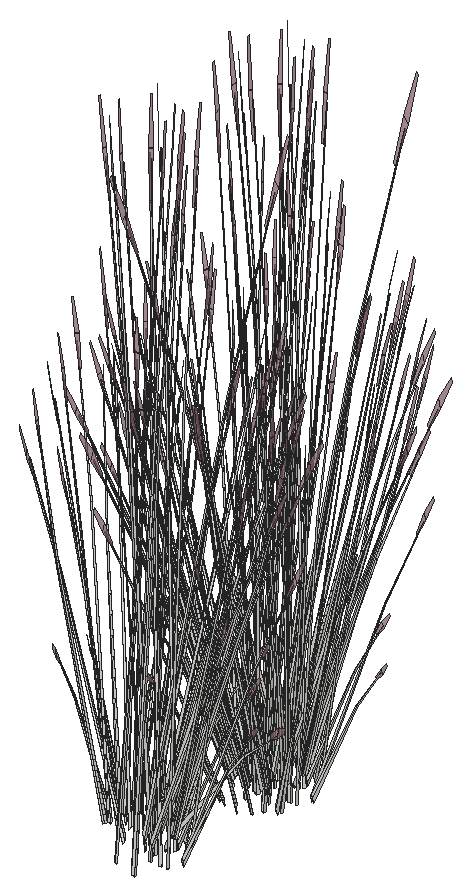
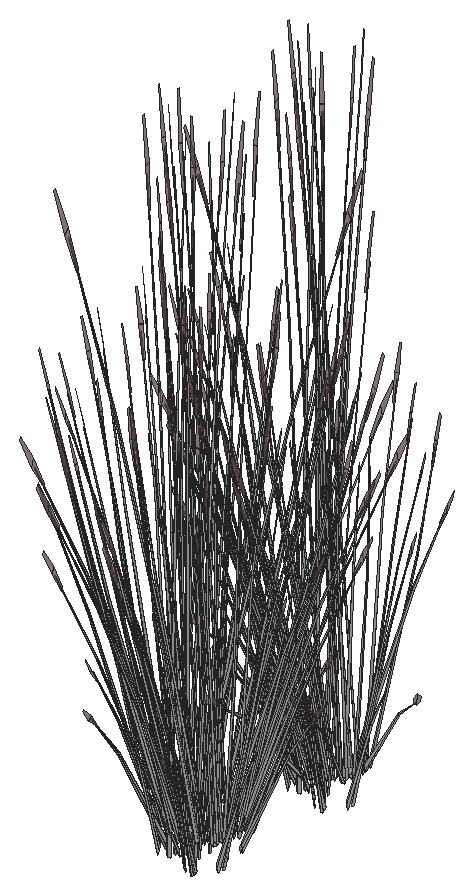
# SketchUp Ruby script. Lengths in inches.
U = 1.inch
M = Sketchup.active_model
def pt(a) = Geom::Point3d.new(a.map { |v| v * U })
def face(e, loops, mat)
  f = e.add_face(loops[0].map { |a| pt(a) })
  loops[1..].each { |l| e.add_face(l.map { |a| pt(a) }).erase! }
  f.material = f.back_material = mat if mat
  f
end
# faces: each face lists its corners as indices into pts; further lists are holes
def faces(e, pts, list, mat = nil) = list.each { |f| face(e, (f[0].is_a?(Array) ? f : [f]).map { |l| l.map { |i| pts[i] } }, mat) }
# xy, xz, yz: faces in a plane at the given z, y or x. An outline is a flat list of corners, or four numbers for a rectangle; further outlines are holes
def ring(l) = l.size == 4 ? [[l[0], l[1]], [l[2], l[1]], [l[2], l[3]], [l[0], l[3]]] : l.each_slice(2).to_a
def flat(e, list, mat, &to3) = list.each { |f| face(e, (f[0].is_a?(Array) ? f : [f]).map { |l| ring(l).map { |u, v| to3.(u, v) } }, mat) }
def xy(e, z, list, mat = nil) = flat(e, list, mat) { |x, y| [x, y, z] }
def xz(e, y, list, mat = nil) = flat(e, list, mat) { |x, z| [x, y, z] }
def yz(e, x, list, mat = nil) = flat(e, list, mat) { |y, z| [x, y, z] }
def lines(e, pts, list) = list.each { |a, b| e.add_line(pt(pts[a]), pt(pts[b])) }
# prism: a flat outline (further loops are holes) pulled along v
def prism(e, loops, v, mat = nil)
  f = face(e, loops, mat); d = Geom::Vector3d.new(v.map { |x| x * U })
  f.pushpull(f.normal.samedirection?(d) ? d.length : -d.length)
end
def box(e, o, s, mat = nil) = prism(e, [[o, [o[0] + s[0], o[1], o[2]], [o[0] + s[0], o[1] + s[1], o[2]], [o[0], o[1] + s[1], o[2]]]], [0, 0, s[2]], mat)
def at(x, y, z, deg = 0) = Geom::Transformation.translation(pt([x, y, z])) * Geom::Transformation.rotation(ORIGIN, Z_AXIS, deg.degrees)
def axes(o, x, y, z) = Geom::Transformation.new([*x, 0, *y, 0, *z, 0, *pt(o).to_a, 1])
def part(name) = M.definitions.add(name)
# library, detail: a bought-in or finely detailed component or shape, given as its bounding box
def library(name, o, s) = part(name).tap { |d| box(d.entities, o, s) }
def detail(e, o, s) = box(e.add_group.entities, o, s)
def put(e, d, t, mat = nil) = e.add_instance(d, t).tap { |i| i.material = mat if mat }
def group(e, t, mat = nil) = e.add_group.tap { |g| g.transformation = t; g.material = mat if mat }.entities
root = M.entities
M.materials.add("LightPink_Translucent").color = [144, 107, 117]
M.materials["LightPink_Translucent"].alpha = 0.75
c1 = part("blade")
p = [[2.15,0.21,22],[0,0.17,0],[0.09,0.45,0],[2.18,0.31,22],[2.29,0.31,22],[0.38,0.45,0],
  [2.48,0.24,33],[2.49,0.24,33],[2.48,0.22,33]]
faces(c1.entities,p,[[0,1,2,3],[4,5,2,3],[6,3,4,7],[8,0,3,6]])
c2 = part("seeds")
p = [[0.3,-0.1,1.38],[-0.01,-0.03,1.59],[-0.01,-0.03,0.03],[0.14,-0.07,-0.07],[0.29,-0.03,3],[0.15,0.01,3.11]]
faces(c2.entities,p,[[0,1,2,3],[1,0,4,5]],"LightPink_Translucent")
c3 = part("blade with seeds")
put(c3.entities,c1,at(0,0,0))
put(c3.entities,c2,axes([2.4,0.25,30.99],[1.5799,-0.05474,1.17369],[-0.12525,1.92788,0.29478],[-0.07173,-0.02425,1.56792]))
put(root,c3,axes([372.04,325.99,152.33],[-0.4583,-0.30184,0.46672],[0.27394,-0.54125,0],[0.10438,0.06875,1.48054]))
put(root,c3,axes([372.94,328.11,154.68],[0.4303,-0.26662,-0.66783],[0.23981,0.54882,0.08059],[0.20791,-0.06234,0.9447]))
put(root,c3,axes([370.31,326.27,152.33],[-0.14146,0.59996,0.16584],[-0.51766,-0.16978,0.32981],[0.08942,-0.00292,1.50782]))
put(root,c3,axes([371.19,327.07,152.56],[-0.29417,-0.5067,0.42055],[0.44558,-0.35681,-0.2024],[0.0952,0.0627,1.35025]))
put(root,c3,axes([370.26,329.36,152.33],[0.52621,-0.16023,0.16584],[0.12993,0.59629,0.32981],[-0.04693,-0.08688,1.50782]))
put(root,c3,axes([373.31,328.16,154.25],[0.40696,0.16841,-0.33289],[-0.1187,0.49132,0.42977],[0.16385,-0.04505,0.82232]))
put(root,c3,axes([368.52,327.38,154.25],[-0.40696,-0.16841,-0.33289],[0.1187,-0.49132,0.42977],[-0.16385,0.04505,0.82232]))
put(root,c3,axes([371.87,326.3,152.33],[-0.52621,0.16023,0.16584],[-0.12993,-0.59629,0.32981],[0.04693,0.08688,1.50782]))
put(root,c3,axes([372.2,327.56,153.64],[-0.20312,0.01367,1.61094],[0.13474,-0.59258,0.13026],[0.28946,0.03665,0.68866]))
put(root,c3,axes([370.74,328.73,152.46],[-0.09447,0.53876,0.13611],[-0.46155,-0.09352,-0.38866],[-0.084,-0.05532,1.1914]))
put(root,c3,axes([371.82,329.39,152.33],[0.14146,-0.59996,0.16584],[0.51766,0.16978,0.32981],[-0.08942,0.00292,1.50782]))
put(root,c3,axes([369.76,327.3,153.14],[0.13919,-0.08733,1.6644],[0.048,0.60974,0.13026],[-0.3015,0.08091,0.59487]))
put(root,c3,axes([372.63,327.86,152.33],[-0.38474,-0.43973,0.16584],[0.38772,-0.42651,0.32981],[-0.04249,0.0898,1.50782]))
put(root,c3,axes([374.17,328.26,152.6],[-0.30256,0.09966,1.07969],[0.14242,-0.41189,0.79328],[0.16051,0.02818,0.23781]))
put(root,c3,axes([370.08,329.66,152.33],[0.4583,0.30184,0.46672],[-0.27394,0.54125,0],[-0.10438,-0.06875,1.48054]))
put(root,c3,axes([371.7,327.58,152.56],[0.23759,-0.54397,0.42055],[0.49367,0.26179,-0.2024],[0,0.12539,1.35025]))
put(root,c3,axes([368.27,327.71,154.43],[-0.07997,0.07838,1.64448],[0.0068,0.57266,-0.26007],[-0.1833,0.07447,0.13189]))
put(root,c3,axes([368.8,327.63,154.4],[-0.13266,0.54912,-0.48033],[-0.45484,-0.18822,-0.37205],[-0.18313,0.05035,0.91906]))
put(root,c3,axes([368.78,327.16,154.73],[0.24639,0.54664,-0.11431],[-0.43729,0.26863,-0.63445],[-0.18428,0.07212,0.96403]))
put(root,c3,axes([373.64,329.53,153.69],[-0.09372,-0.50747,-0.03282],[0.44299,-0.11666,-0.14882],[0.09251,0.03217,0.49085]))
put(root,c3,axes([372.49,329.52,154.73],[0.02622,-0.61393,-0.11431],[0.49645,0.01678,-0.63445],[0.1912,0.04265,0.96403]))
put(root,c3,axes([372.95,327.88,152.33],[0,-0.60368,0.46672],[0.54787,0,0],[0,0.13749,1.48054]))
put(root,c3,axes([371.57,328.33,152.56],[0.53176,-0.03727,0.42055],[0.04809,0.6186,-0.2024],[-0.0952,0.0627,1.35025]))
put(root,c3,axes([373.6,328.92,152.44],[-0.11793,-0.14847,1.34422],[0.15345,-0.49116,-0.28909],[0.23861,0.06653,0.57472]))
put(root,c3,axes([372.93,329.15,154.43],[0.10505,-0.01021,1.64448],[0.28813,-0.469,-0.26007],[0.18685,0.06191,0.13189]))
put(root,c3,axes([368.79,327.92,153.64],[0.16991,-0.12769,1.61094],[0.14304,0.59005,0.13026],[-0.26674,0.13336,0.68866]))
put(root,c3,axes([372.52,329.22,154.68],[0.48951,0.01454,-0.66783],[-0.03288,0.61207,0.08059],[0.20738,0.06459,0.9447]))
put(root,c3,axes([371.97,329.71,152.33],[0.4583,-0.30184,0.46672],[0.27394,0.54125,0],[-0.10438,0.06875,1.48054]))
put(root,c3,axes([368.26,328.92,152.44],[0.17018,0.04956,1.34422],[0.10969,0.50618,-0.28909],[-0.23117,0.09475,0.57472]))
put(root,c3,axes([367.9,329.98,152.6],[0.20408,-0.2736,1.07969],[0.08053,0.43313,0.79328],[-0.14748,0.07756,0.23781]))
put(root,c3,axes([372.8125,329.48,154.25],[0.27863,0.37797,-0.33289],[-0.31815,0.35779,0.42977],[0.16164,0.05444,0.82232]))
put(root,c3,axes([368.67,328.8,154.25],[-0.42626,0.08628,-0.33289],[-0.11256,-0.4932,0.42977],[-0.12215,0.13247,0.82232]))
put(root,c3,axes([371.09,336.94,153.64],[0.11194,0.19382,1.61094],[-0.51725,0.16318,0.13026],[-0.1169,-0.30428,0.68866]))
put(root,c3,axes([371.8125,328.51,153.64],[-0.1819,-0.10401,1.61094],[0.37643,-0.43634,0.13026],[0.23461,0.19684,0.68866]))
put(root,c3,axes([371.85,327.14,154.21],[-0.42314,-0.31366,1.29986],[0.4468,-0.48836,0.56085],[0.13652,0.29431,1.25644]))
put(root,c3,axes([373.11,336.66,152.44],[-0.13919,0.12219,1.34422],[-0.41687,-0.21387,-0.28909],[0.07727,-0.26598,0.57472]))
put(root,c3,axes([372.47,337.09,154.68],[-0.23372,-0.49086,-0.66783],[0.48111,-0.27356,0.08059],[-0.05465,-0.23717,0.9447]))
put(root,c3,axes([368.8,328.46,154.73],[0.45297,0.33287,-0.11431],[-0.26096,0.48206,-0.63445],[-0.12798,0.16757,0.96403]))
put(root,c3,axes([372.49,329.69,152.6],[-0.27572,-0.17358,1.07969],[0.35602,-0.17637,0.79328],[0.09603,0.1494,0.23781]))
put(root,c3,axes([370.95,336.43,152.44],[-0.02965,0.19748,1.34422],[-0.43351,0.16532,-0.28909],[-0.10133,-0.25525,0.57472]))
put(root,c3,axes([371.52,330.1875,154.73],[0.2918,-0.51673,-0.11431],[0.42258,0.29769,-0.63445],[0.14689,0.14599,0.96403]))
put(root,c3,axes([369.41,328.3125,153.64],[0.12231,-0.18549,1.61094],[0.30882,0.50067,0.13026],[-0.21182,0.22801,0.68866]))
put(root,c3,axes([369.02,328.86,154.4],[0.1258,0.55122,-0.48033],[-0.4764,0.09643,-0.37205],[-0.13652,0.14806,0.91906]))
put(root,c3,axes([373.45,337.57,154.68],[0.01274,-0.55841,-0.66783],[0.53656,0.0375,0.08059],[0.05662,-0.23657,0.9447]))
put(root,c3,axes([371.81,327.74,152.67],[-0.01338,-0.56839,1.32796],[0.60542,0.14734,0.56227],[-0.14319,0.31102,1.25349]))
put(root,c3,axes([372.52,336.67,154.25],[0.14763,-0.46424,-0.33289],[0.4307,0.1354,0.42977],[-0.03949,-0.18691,0.82232]))
put(root,c3,axes([372.84,337.29,153.64],[-0.09118,0.2075,1.61094],[-0.3825,-0.42941,0.13026],[0.17255,-0.26763,0.68866]))
put(root,c3,axes([371.86,329.93,154.4],[0.48321,-0.1435,-0.48033],[0.08453,0.54345,-0.37205],[0.12979,0.15574,0.91906]))
put(root,c3,axes([372.3,336.99,154.4],[-0.48137,-0.15133,-0.48033],[0.165,-0.51886,-0.37205],[-0.04414,-0.2089,0.91906]))
put(root,c3,axes([372.59,335.69,152.6],[0.06282,0.35202,1.07969],[-0.34848,-0.19497,0.79328],[0.0375,-0.18025,0.23781]))
put(root,c3,axes([372.53,330.48,152.51],[-0.31402,-0.01893,0.98757],[0.20738,-0.40212,0.54525],[0.12405,0.14286,0.77466]))
put(root,c3,axes([373.34,337.38,154.4],[-0.35055,-0.40562,-0.48033],[0.37031,-0.35523,-0.37205],[0.05334,-0.20609,0.91906]))
put(root,c3,axes([369.32,328.77,153.64],[0.09118,-0.2075,1.61094],[0.3825,0.42941,0.13026],[-0.17255,0.26763,0.68866]))
put(root,c3,axes([372.71,336.97,154.73],[-0.47919,0.28106,-0.11431],[-0.23549,-0.49884,-0.63445],[-0.06322,-0.21021,0.96403]))
put(root,c3,axes([373.7,337.6,154.73],[-0.53819,-0.02991,-0.11431],[0.01471,-0.56632,-0.63445],[0.03738,-0.21811,0.96403]))
put(root,c3,axes([371.5,329.51,152.44],[0.00864,-0.20012,1.34422],[0.41296,-0.22353,-0.28909],[0.12748,0.23952,0.57472]))
put(root,c3,axes([373.67,337.23,154.25],[0.33133,-0.31784,-0.33289],[0.31365,0.36292,0.42977],[0.04772,-0.1844,0.82232]))
put(root,c3,axes([370.8,336.11,152.6],[0.25544,0.21011,1.07969],[-0.37201,0.1263,0.79328],[-0.0796,-0.16148,0.23781]))
put(root,c3,axes([371.42,337.23,154.68],[-0.41756,-0.29179,-0.66783],[0.29675,-0.51132,0.08059],[-0.15128,-0.17422,0.9447]))
put(root,c3,axes([371.28,336.84,154.25],[-0.07563,-0.48625,-0.33289],[0.43235,-0.1284,0.42977],[-0.11613,-0.13934,0.82232]))
put(root,c3,axes([369.42,329.94,154.25],[-0.33133,0.31784,-0.33289],[-0.31365,-0.36292,0.42977],[-0.04772,0.1844,0.82232]))
put(root,c3,axes([368.28,329.85,154.43],[-0.01217,0.11946,1.64448],[0.34544,0.41559,-0.26007],[-0.09043,0.19653,0.13189]))
put(root,c3,axes([370.38,330.21,154.73],[0.47919,-0.28106,-0.11431],[0.23549,0.49884,-0.63445],[0.06322,0.21021,0.96403]))
put(root,c3,axes([369.63,331.17,152.6],[-0.01267,-0.35895,1.07969],[0.31667,0.25602,0.79328],[-0.06228,0.17109,0.23781]))
put(root,c3,axes([369.75,329.79,154.7],[0.35055,0.40562,-0.53317],[-0.37031,0.35523,-0.41298],[-0.05334,0.20609,1.02016]))
put(root,c3,axes([370.34,337.55,153.64],[0.1819,0.10401,1.61094],[-0.37643,0.43634,0.13026],[-0.23461,-0.19684,0.68866]))
put(root,c3,axes([369.37,330.4,152.65],[0.44486,-0.1069,0.06117],[0.10227,0.43069,-0.81126],[-0.0282,0.21802,0.72719]))
put(root,c3,axes([370.79,330.18,154.4],[0.48137,0.15133,-0.48033],[-0.165,0.51886,-0.37205],[0.04414,0.2089,0.91906]))
put(root,c3,axes([371.0625,329.11,153.64],[-0.11194,-0.19382,1.61094],[0.51725,-0.16318,0.13026],[0.1169,0.30428,0.68866]))
put(root,c3,axes([371.22,337.24,154.4],[-0.48321,0.1435,-0.48033],[-0.08453,-0.54345,-0.37205],[-0.12979,-0.15574,0.91906]))
put(root,c3,axes([370.57,330.5,154.25],[-0.14763,0.46424,-0.33289],[-0.4307,-0.1354,0.42977],[0.03949,0.18691,0.82232]))
put(root,c3,axes([369.64,329.6,155.02],[-0.01274,0.55841,-0.74129],[-0.53656,-0.0375,0.08946],[-0.05662,0.23657,1.04862]))
put(root,c3,axes([374.08,338.54,154.68],[0.25579,-0.47633,-0.66783],[0.44823,0.33852,0.08059],[0.15273,-0.17258,0.9447]))
put(root,c3,axes([374.07,338.32,154.4],[-0.1258,-0.55122,-0.48033],[0.4764,-0.09643,-0.37205],[0.13652,-0.14806,0.91906]))
put(root,c3,axes([370.15,329.21,153.64],[-0.01199,-0.2317,1.61094],[0.51947,0.15371,0.13026],[-0.03213,0.3302,0.68866]))
put(root,c3,axes([374.29,338.71,154.73],[-0.45297,-0.33287,-0.11431],[0.26096,-0.48206,-0.63445],[0.12798,-0.16757,0.96403]))
put(root,c3,axes([370.62,330.08,154.68],[0.23372,0.49086,-0.66783],[-0.48111,0.27356,0.08059],[0.05465,0.23717,0.9447]))
put(root,c3,axes([369.26,330.86,152.44],[0.15453,-0.09523,1.34422],[0.38153,0.28715,-0.28909],[-0.11356,0.24846,0.57472]))
put(root,c3,axes([370.27,331.32,154.43],[0.06207,0.09721,1.64448],[0.50093,0.03819,-0.26007],[0.05037,0.21439,0.13189]))
put(root,c3,axes([372.42,340.53,153.125],[0.42317,0.24343,1.42185],[-0.41456,0.52443,0.56227],[-0.18569,-0.31082,1.19198]))
put(root,c3,axes([374.45,338.1,152.44],[-0.17494,-0.01788,1.34422],[-0.17922,-0.47967,-0.28909],[0.21491,-0.13569,0.57472]))
put(root,c3,axes([374.65,337.22,152.6],[-0.16311,0.3073,1.07969],[-0.1402,-0.41288,0.79328],[0.13471,-0.10346,0.23781]))
put(root,c3,axes([374.42,338.375,154.25],[0.42626,-0.08628,-0.33289],[0.11256,0.4932,0.42977],[0.12215,-0.13247,0.82232]))
put(root,c3,axes([369.46,330.39,153.16],[0.01076,-0.31164,1.45085],[0.48391,0.16461,0.20049],[-0.04193,0.33214,0.68509]))
put(root,c3,axes([370.27,337.7,154.25],[-0.27863,-0.37797,-0.33289],[0.31815,-0.35779,0.42977],[-0.16164,-0.05444,0.82232]))
put(root,c3,axes([370.17,338.1,152.44],[0.09561,0.16807,1.34422],[-0.22031,0.45686,-0.28909],[-0.22622,-0.1092,0.57472]))
put(root,c3,axes([370.57,337.95,154.68],[-0.48951,-0.01454,-0.66783],[0.03288,-0.61207,0.08059],[-0.20738,-0.06459,0.9447]))
put(root,c3,axes([370.41,338.07,154.4],[-0.35558,0.39989,-0.48033],[-0.31141,-0.42243,-0.37205],[-0.18066,-0.06084,0.91906]))
put(root,c3,axes([369.61,338.6,152.6],[0.31263,-0.0432,1.07969],[-0.19831,0.38061,0.79328],[-0.15449,-0.0571,0.23781]))
put(root,c3,axes([371.8125,338.96,152.56],[-0.53176,0.03727,0.42055],[-0.04809,-0.6186,-0.2024],[0.0952,-0.0627,1.35025]))
put(root,c3,axes([370.59,337.65,154.73],[-0.02622,0.61393,-0.11431],[-0.49645,-0.01678,-0.63445],[-0.1912,-0.04265,0.96403]))
put(root,c3,axes([370.44,339.41,152.33],[0,0.60368,0.46672],[-0.54787,0,0],[0,-0.13749,1.48054]))
put(root,c3,axes([374.31,340.01,154.73],[-0.24639,-0.54664,-0.11431],[0.43729,-0.26863,-0.63445],[0.18428,-0.07212,0.96403]))
put(root,c3,axes([374.29,339.54,154.4],[0.13266,-0.54912,-0.48033],[0.45484,0.18822,-0.37205],[0.18313,-0.05035,0.91906]))
put(root,c3,axes([369.96,338.5,153.64],[0.20312,-0.01367,1.61094],[-0.13474,0.59258,0.13026],[-0.28946,-0.03665,0.68866]))
put(root,c3,axes([371.6875,339.71,152.56],[-0.23759,0.54397,0.42055],[-0.49367,-0.26179,-0.2024],[0,-0.12539,1.35025]))
put(root,c3,axes([373.3,337.62,152.33],[-0.4583,-0.30184,0.46672],[0.27394,-0.54125,0],[0.10438,0.06875,1.48054]))
put(root,c3,axes([374.2,339.74,154.68],[0.4303,-0.26662,-0.66783],[0.23981,0.54882,0.08059],[0.20791,-0.06234,0.9447]))
put(root,c3,axes([371.57,337.89,152.33],[-0.14146,0.59996,0.16584],[-0.51766,-0.16978,0.32981],[0.08942,-0.00292,1.50782]))
put(root,c3,axes([372.65,338.5625,152.46],[0.09447,-0.53876,0.13611],[0.46155,0.09352,-0.38866],[0.084,0.05532,1.1914]))
put(root,c3,axes([372.45,338.7,152.56],[-0.29417,-0.5067,0.42055],[0.44558,-0.35681,-0.2024],[0.0952,0.0627,1.35025]))
put(root,c3,axes([371.52,340.99,152.33],[0.52621,-0.16023,0.16584],[0.12993,0.59629,0.32981],[-0.04693,-0.08688,1.50782]))
put(root,c3,axes([374.57,339.79,154.25],[0.40696,0.16841,-0.33289],[-0.1187,0.49132,0.42977],[0.16385,-0.04505,0.82232]))
put(root,c3,axes([369.78,339.01,154.25],[-0.40696,-0.16841,-0.33289],[0.1187,-0.49132,0.42977],[-0.16385,0.04505,0.82232]))
put(root,c3,axes([373.13,337.93,152.33],[-0.52621,0.16023,0.16584],[-0.12993,-0.59629,0.32981],[0.04693,0.08688,1.50782]))
put(root,c3,axes([373.46,339.18,153.64],[-0.20312,0.01367,1.61094],[0.13474,-0.59258,0.13026],[0.28946,0.03665,0.68866]))
put(root,c3,axes([372,340.35,152.46],[-0.09447,0.53876,0.13611],[-0.46155,-0.09352,-0.38866],[-0.084,-0.05532,1.1914]))
put(root,c3,axes([373.08,341.02,152.33],[0.14146,-0.59996,0.16584],[0.51766,0.16978,0.32981],[-0.08942,0.00292,1.50782]))
put(root,c3,axes([371.02,338.93,153.14],[0.13919,-0.08733,1.6644],[0.048,0.60974,0.13026],[-0.3015,0.08091,0.59487]))
put(root,c3,axes([373.89,339.49,152.33],[-0.38474,-0.43973,0.16584],[0.38772,-0.42651,0.32981],[-0.04249,0.0898,1.50782]))
put(root,c3,axes([375.43,339.89,152.6],[-0.30256,0.09966,1.07969],[0.14242,-0.41189,0.79328],[0.16051,0.02818,0.23781]))
put(root,c3,axes([371.35,341.29,152.33],[0.4583,0.30184,0.46672],[-0.27394,0.54125,0],[-0.10438,-0.06875,1.48054]))
put(root,c3,axes([372.96,339.2,152.56],[0.23759,-0.54397,0.42055],[0.49367,0.26179,-0.2024],[0,0.12539,1.35025]))
put(root,c3,axes([370.0625,339.26,154.4],[-0.13266,0.54912,-0.48033],[-0.45484,-0.18822,-0.37205],[-0.18313,0.05035,0.91906]))
put(root,c3,axes([370.04,338.79,154.73],[0.24639,0.54664,-0.11431],[-0.43729,0.26863,-0.63445],[-0.18428,0.07212,0.96403]))
put(root,c3,axes([374.9,341.16,153.69],[-0.09372,-0.50747,-0.03282],[0.44299,-0.11666,-0.14882],[0.09251,0.03217,0.49085]))
put(root,c3,axes([373.75,341.15,154.73],[0.02622,-0.61393,-0.11431],[0.49645,0.01678,-0.63445],[0.1912,0.04265,0.96403]))
put(root,c3,axes([374.21,339.51,152.33],[0,-0.60368,0.46672],[0.54787,0,0],[0,0.13749,1.48054]))
put(root,c3,axes([372.83,339.96,152.56],[0.53176,-0.03727,0.42055],[0.04809,0.6186,-0.2024],[-0.0952,0.0627,1.35025]))
put(root,c3,axes([373.17,339.33,152.46],[0.45625,-0.17605,0.13611],[0.15978,0.50273,-0.38866],[0,0.11064,1.1914]))
put(root,c3,axes([374.86,340.55,152.44],[-0.11793,-0.14847,1.34422],[0.15345,-0.49116,-0.28909],[0.23861,0.06653,0.57472]))
put(root,c3,axes([372.84,340.22,152.46],[0.36178,0.36271,0.13611],[-0.30177,0.40921,-0.38866],[-0.084,0.05532,1.1914]))
put(root,c3,axes([370.05,339.54,153.64],[0.16991,-0.12769,1.61094],[0.14304,0.59005,0.13026],[-0.26674,0.13336,0.68866]))
put(root,c3,axes([373.78,340.85,154.68],[0.48951,0.01454,-0.66783],[-0.03288,0.61207,0.08059],[0.20738,0.06459,0.9447]))
put(root,c3,axes([373.23,341.34,152.33],[0.4583,-0.30184,0.46672],[0.27394,0.54125,0],[-0.10438,0.06875,1.48054]))
put(root,c3,axes([369.52,340.55,152.44],[0.17018,0.04956,1.34422],[0.10969,0.50618,-0.28909],[-0.23117,0.09475,0.57472]))
put(root,c3,axes([369.16,341.61,152.6],[0.20408,-0.2736,1.07969],[0.08053,0.43313,0.79328],[-0.14748,0.07756,0.23781]))
put(root,c3,axes([374.07,341.1,154.25],[0.27863,0.37797,-0.33289],[-0.31815,0.35779,0.42977],[0.16164,0.05444,0.82232]))
put(root,c3,axes([369.93,340.43,154.25],[-0.42626,0.08628,-0.33289],[-0.11256,-0.4932,0.42977],[-0.12215,0.13247,0.82232]))
put(root,c3,axes([373.07,340.14,153.64],[-0.1819,-0.10401,1.61094],[0.37643,-0.43634,0.13026],[0.23461,0.19684,0.68866]))
put(root,c3,axes([373.11,338.77,154.21],[-0.42314,-0.31366,1.29986],[0.4468,-0.48836,0.56085],[0.13652,0.29431,1.25644]))
put(root,c3,axes([370.06,340.09,154.73],[0.45297,0.33287,-0.11431],[-0.26096,0.48206,-0.63445],[-0.12798,0.16757,0.96403]))
put(root,c3,axes([373.75,341.32,152.6],[-0.27572,-0.17358,1.07969],[0.35602,-0.17637,0.79328],[0.09603,0.1494,0.23781]))
put(root,c3,axes([372.78,341.81,154.73],[0.2918,-0.51673,-0.11431],[0.42258,0.29769,-0.63445],[0.14689,0.14599,0.96403]))
put(root,c3,axes([370.67,339.94,153.64],[0.12231,-0.18549,1.61094],[0.30882,0.50067,0.13026],[-0.21182,0.22801,0.68866]))
put(root,c3,axes([370.28,340.48,154.4],[0.1258,0.55122,-0.48033],[-0.4764,0.09643,-0.37205],[-0.13652,0.14806,0.91906]))
put(root,c3,axes([373.07,339.37,152.67],[-0.01338,-0.56839,1.32796],[0.60542,0.14734,0.56227],[-0.14319,0.31102,1.25349]))
put(root,c3,axes([373.125,341.56,154.4],[0.48321,-0.1435,-0.48033],[0.08453,0.54345,-0.37205],[0.12979,0.15574,0.91906]))
put(root,c3,axes([373.79,342.11,152.51],[-0.31402,-0.01893,0.98757],[0.20738,-0.40212,0.54525],[0.12405,0.14286,0.77466]))
put(root,c3,axes([370.58,340.4,153.64],[0.09118,-0.2075,1.61094],[0.3825,0.42941,0.13026],[-0.17255,0.26763,0.68866]))
put(root,c3,axes([372.77,341.13,152.44],[0.00864,-0.20012,1.34422],[0.41296,-0.22353,-0.28909],[0.12748,0.23952,0.57472]))
put(root,c3,axes([370.68,341.57,154.25],[-0.33133,0.31784,-0.33289],[-0.31365,-0.36292,0.42977],[-0.04772,0.1844,0.82232]))
put(root,c3,axes([371.64,341.84,154.73],[0.47919,-0.28106,-0.11431],[0.23549,0.49884,-0.63445],[0.06322,0.21021,0.96403]))
put(root,c3,axes([370.89,342.8,152.6],[-0.01267,-0.35895,1.07969],[0.31667,0.25602,0.79328],[-0.06228,0.17109,0.23781]))
put(root,c3,axes([371.01,341.42,154.7],[0.35055,0.40562,-0.53317],[-0.37031,0.35523,-0.41298],[-0.05334,0.20609,1.02016]))
put(root,c3,axes([370.63,342.03,152.65],[0.44486,-0.1069,0.06117],[0.10227,0.43069,-0.81126],[-0.0282,0.21802,0.72719]))
put(root,c3,axes([372.05,341.8125,154.4],[0.48137,0.15133,-0.48033],[-0.165,0.51886,-0.37205],[0.04414,0.2089,0.91906]))
put(root,c3,axes([372.32,340.74,153.64],[-0.11194,-0.19382,1.61094],[0.51725,-0.16318,0.13026],[0.1169,0.30428,0.68866]))
put(root,c3,axes([371.83,342.13,154.25],[-0.14763,0.46424,-0.33289],[-0.4307,-0.1354,0.42977],[0.03949,0.18691,0.82232]))
put(root,c3,axes([370.9,341.23,155.02],[-0.01274,0.55841,-0.74129],[-0.53656,-0.0375,0.08946],[-0.05662,0.23657,1.04862]))
put(root,c3,axes([371.41,340.84,153.64],[-0.01199,-0.2317,1.61094],[0.51947,0.15371,0.13026],[-0.03213,0.3302,0.68866]))
put(root,c3,axes([371.875,341.71,154.68],[0.23372,0.49086,-0.66783],[-0.48111,0.27356,0.08059],[0.05465,0.23717,0.9447]))
put(root,c3,axes([370.52,342.48,152.44],[0.15453,-0.09523,1.34422],[0.38153,0.28715,-0.28909],[-0.11356,0.24846,0.57472]))
put(root,c3,axes([370.72,342.02,153.16],[0.01076,-0.31164,1.45085],[0.48391,0.16461,0.20049],[-0.04193,0.33214,0.68509]))
